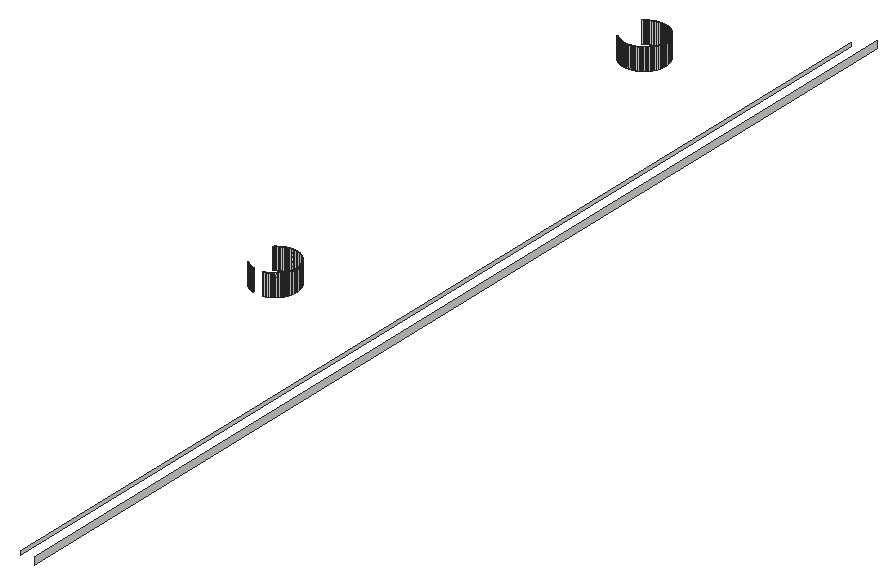
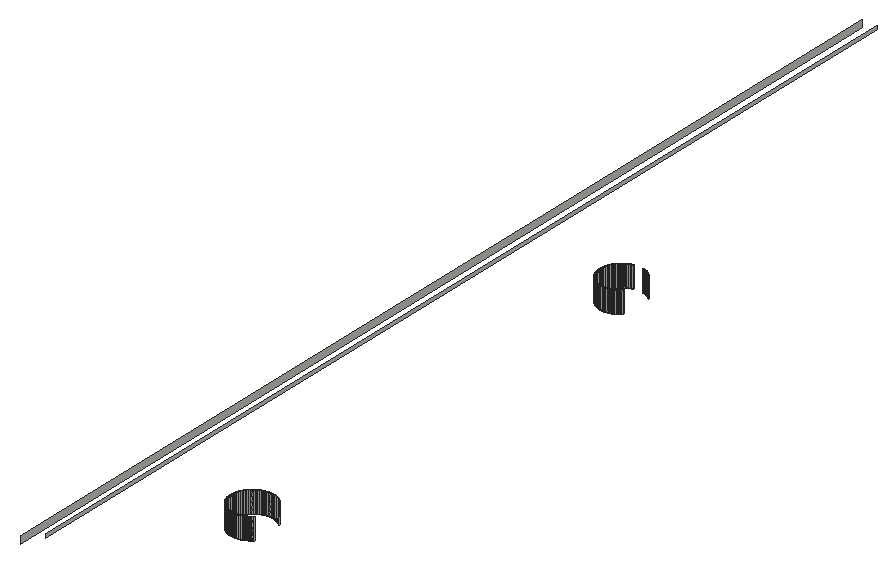
# SketchUp Ruby script. Lengths in inches.
U = 1.inch
M = Sketchup.active_model
def pt(a) = Geom::Point3d.new(a.map { |v| v * U })
def face(e, loops, mat)
  f = e.add_face(loops[0].map { |a| pt(a) })
  loops[1..].each { |l| e.add_face(l.map { |a| pt(a) }).erase! }
  f.material = f.back_material = mat if mat
  f
end
# faces: each face lists its corners as indices into pts; further lists are holes
def faces(e, pts, list, mat = nil) = list.each { |f| face(e, (f[0].is_a?(Array) ? f : [f]).map { |l| l.map { |i| pts[i] } }, mat) }
# xy, xz, yz: faces in a plane at the given z, y or x. An outline is a flat list of corners, or four numbers for a rectangle; further outlines are holes
def ring(l) = l.size == 4 ? [[l[0], l[1]], [l[2], l[1]], [l[2], l[3]], [l[0], l[3]]] : l.each_slice(2).to_a
def flat(e, list, mat, &to3) = list.each { |f| face(e, (f[0].is_a?(Array) ? f : [f]).map { |l| ring(l).map { |u, v| to3.(u, v) } }, mat) }
def xy(e, z, list, mat = nil) = flat(e, list, mat) { |x, y| [x, y, z] }
def xz(e, y, list, mat = nil) = flat(e, list, mat) { |x, z| [x, y, z] }
def yz(e, x, list, mat = nil) = flat(e, list, mat) { |y, z| [x, y, z] }
def lines(e, pts, list) = list.each { |a, b| e.add_line(pt(pts[a]), pt(pts[b])) }
# prism: a flat outline (further loops are holes) pulled along v
def prism(e, loops, v, mat = nil)
  f = face(e, loops, mat); d = Geom::Vector3d.new(v.map { |x| x * U })
  f.pushpull(f.normal.samedirection?(d) ? d.length : -d.length)
end
def box(e, o, s, mat = nil) = prism(e, [[o, [o[0] + s[0], o[1], o[2]], [o[0] + s[0], o[1] + s[1], o[2]], [o[0], o[1] + s[1], o[2]]]], [0, 0, s[2]], mat)
def at(x, y, z, deg = 0) = Geom::Transformation.translation(pt([x, y, z])) * Geom::Transformation.rotation(ORIGIN, Z_AXIS, deg.degrees)
def axes(o, x, y, z) = Geom::Transformation.new([*x, 0, *y, 0, *z, 0, *pt(o).to_a, 1])
def part(name) = M.definitions.add(name)
# library, detail: a bought-in or finely detailed component or shape, given as its bounding box
def library(name, o, s) = part(name).tap { |d| box(d.entities, o, s) }
def detail(e, o, s) = box(e.add_group.entities, o, s)
def put(e, d, t, mat = nil) = e.add_instance(d, t).tap { |i| i.material = mat if mat }
def group(e, t, mat = nil) = e.add_group.tap { |g| g.transformation = t; g.material = mat if mat }.entities
root = M.entities
xz(root,255.5,[[328.84,108,328.92,111],[328.92,108,329,111],[329,108,329.08,111],[329.08,108,329.16,111]])
xz(root,314,[[328.84,108,328.92,111],[328.92,108,329,111],[329,108,329.08,111],[329.08,108,329.16,111]])
xz(root,320,[[328.84,108,328.92,111],[328.92,108,329,111],[329,108,329.08,111],[329.08,108,329.16,111]])
yz(root,332,[[252.34,108,252.42,111],[252.42,108,252.5,111],[252.5,108,252.58,111],[252.58,108,252.66,111],[316.84,108,316.92,111],
  [316.92,108,317,111],[317,108,317.08,111],[317.08,108,317.16,111]])
yz(root,345,[[187.96,108,333,108.5]])
yz(root,347,[[187.97,107.5,335,108.5]])
p = [[328.07,249.65,108],[328,249.67,108],[328,249.67,111],[328.07,249.65,111],[328.15,249.625,108],[328.15,249.625,111],
  [328.22,249.6,108],[328.22,249.6,111],[328.3,249.58,108],[328.3,249.58,111],[328.375,249.57,108],[328.375,249.57,111],
  [329.625,249.57,108],[329.55,249.55,108],[329.55,249.55,111],[329.625,249.57,111],[329.7,249.58,108],[329.7,249.58,111],
  [329.78,249.6,108],[329.78,249.6,111],[329.85,249.625,108],[329.85,249.625,111],[329.93,249.65,108],[329.93,249.65,111],
  [330,249.67,108],[330,249.67,111],[327.85,249.73,108],[327.78,249.76,108],[327.78,249.76,111],[327.85,249.73,111],
  [327.92,249.7,108],[327.92,249.7,111],[330.08,249.7,108],[330.08,249.7,111],[330.15,249.73,108],[330.15,249.73,111],
  [330.22,249.76,108],[330.22,249.76,111],[327.64,249.83,108],[327.57,249.86,108],[327.57,249.86,111],[327.64,249.83,111],
  [327.71,249.79,108],[327.71,249.79,111],[330.29,249.79,108],[330.29,249.79,111],[330.36,249.83,108],[330.36,249.83,111],
  [330.43,249.86,108],[330.43,249.86,111],[327.43,249.94,108],[327.37,249.98,108],[327.37,249.98,111],[327.43,249.94,111],
  [327.5,249.9,108],[327.5,249.9,111],[330.5,249.9,108],[330.5,249.9,111],[330.57,249.94,108],[330.57,249.94,111],
  [330.63,249.98,108],[330.63,249.98,111],[327.3,250.03,108],[327.24,250.07,108],[327.24,250.07,111],[327.3,250.03,111],
  [330.7,250.03,108],[330.7,250.03,111],[330.76,250.07,108],[330.76,250.07,111],[327.17,250.12,108],[327.11,250.17,108],
  [327.11,250.17,111],[327.17,250.12,111],[330.83,250.12,108],[330.83,250.12,111],[330.89,250.17,108],[330.89,250.17,111],
  [327.05,250.22,108],[326.99,250.27,108],[326.99,250.27,111],[327.05,250.22,111],[330.95,250.22,108],[330.95,250.22,111],
  [331.01,250.27,108],[331.01,250.27,111],[326.93,250.32,108],[326.93,250.32,111],[331.07,250.32,108],[331.07,250.32,111],
  [331.12,250.38,108],[331.12,250.38,111],[331.18,250.43,108],[331.18,250.43,111],[331.23,250.49,108],[331.23,250.49,111],
  [331.28,250.55,108],[331.28,250.55,111],[331.33,250.61,108],[331.33,250.61,111],[331.38,250.67,108],[331.38,250.67,111],
  [331.43,250.74,108],[331.43,250.74,111],[331.47,250.8,108],[331.47,250.8,111],[331.52,250.87,108],[331.52,250.87,111],
  [331.56,250.93,108],[331.56,250.93,111],[331.6,251,108],[331.6,251,111],[331.64,251.07,108],[331.64,251.07,111],
  [331.67,251.14,108],[331.67,251.14,111],[331.71,251.21,108],[331.71,251.21,111],[331.74,251.28,108],[331.74,251.28,111],
  [331.77,251.35,108],[331.77,251.35,111],[331.8,251.42,108],[331.8,251.42,111],[331.83,251.5,108],[331.83,251.5,111],
  [331.85,251.57,108],[331.85,251.57,111],[331.875,251.65,108],[331.875,251.65,111],[331.9,251.72,108],[331.9,251.72,111],
  [331.92,251.8,108],[331.92,251.8,111],[331.93,251.875,108],[331.93,251.875,111],[331.95,251.95,108],[331.95,251.95,111],
  [331.96,252.03,108],[331.96,252.03,111],[331.97,252.11,108],[331.97,252.11,111],[331.98,252.1875,108],[331.98,252.1875,111],
  [331.99,252.26,108],[331.99,252.26,111],[332,252.34,108],[332,252.34,111],[331.98,252.8125,108],[331.99,252.74,108],
  [331.99,252.74,111],[331.98,252.8125,111],[332,252.66,108],[332,252.66,111],[331.97,252.89,108],[331.97,252.89,111],
  [331.96,252.97,108],[331.96,252.97,111],[331.93,253.125,108],[331.95,253.05,108],[331.95,253.05,111],[331.93,253.125,111],
  [331.92,253.2,108],[331.92,253.2,111],[331.9,253.28,108],[331.9,253.28,111],[331.875,253.35,108],[331.875,253.35,111],
  [331.83,253.5,108],[331.85,253.43,108],[331.85,253.43,111],[331.83,253.5,111],[331.8,253.58,108],[331.8,253.58,111],
  [331.74,253.72,108],[331.77,253.65,108],[331.77,253.65,111],[331.74,253.72,111],[331.71,253.79,108],[331.71,253.79,111],
  [331.67,253.86,108],[331.67,253.86,111],[331.6,254,108],[331.64,253.93,108],[331.64,253.93,111],[331.6,254,111],
  [331.56,254.07,108],[331.56,254.07,111],[331.47,254.2,108],[331.52,254.13,108],[331.52,254.13,111],[331.47,254.2,111],
  [331.43,254.26,108],[331.43,254.26,111],[331.33,254.39,108],[331.38,254.33,108],[331.38,254.33,111],[331.33,254.39,111],
  [331.23,254.51,108],[331.28,254.45,108],[331.28,254.45,111],[331.23,254.51,111],[331.18,254.57,108],[331.18,254.57,111],
  [331.07,254.68,108],[331.12,254.62,108],[331.12,254.62,111],[331.07,254.68,111],[326.93,254.68,108],[326.99,254.73,108],
  [326.99,254.73,111],[326.93,254.68,111],[327.05,254.78,108],[327.05,254.78,111],[330.95,254.78,108],[331.01,254.73,108],
  [331.01,254.73,111],[330.95,254.78,111],[327.11,254.83,108],[327.11,254.83,111],[327.17,254.88,108],[327.17,254.88,111],
  [330.83,254.88,108],[330.89,254.83,108],[330.89,254.83,111],[330.83,254.88,111],[327.24,254.93,108],[327.24,254.93,111],
  [327.3,254.97,108],[327.3,254.97,111],[330.7,254.97,108],[330.76,254.93,108],[330.76,254.93,111],[330.7,254.97,111],
  [327.37,255.02,108],[327.37,255.02,111],[327.43,255.06,108],[327.43,255.06,111],[330.57,255.06,108],[330.63,255.02,108],
  [330.63,255.02,111],[330.57,255.06,111],[327.5,255.1,108],[327.5,255.1,111],[327.57,255.14,108],[327.57,255.14,111],
  [327.64,255.17,108],[327.64,255.17,111],[330.36,255.17,108],[330.43,255.14,108],[330.43,255.14,111],[330.36,255.17,111],
  [330.5,255.1,108],[330.5,255.1,111],[327.71,255.21,108],[327.71,255.21,111],[327.78,255.24,108],[327.78,255.24,111],
  [327.85,255.27,108],[327.85,255.27,111],[330.15,255.27,108],[330.22,255.24,108],[330.22,255.24,111],[330.15,255.27,111],
  [330.29,255.21,108],[330.29,255.21,111],[327.92,255.3,108],[327.92,255.3,111],[328,255.33,108],[328,255.33,111],
  [328.07,255.35,108],[328.07,255.35,111],[329.93,255.35,108],[330,255.33,108],[330,255.33,111],[329.93,255.35,111],
  [330.08,255.3,108],[330.08,255.3,111],[328.15,255.375,108],[328.15,255.375,111],[328.22,255.4,108],[328.22,255.4,111],
  [328.3,255.42,108],[328.3,255.42,111],[328.375,255.43,108],[328.375,255.43,111],[328.45,255.45,108],[328.45,255.45,111],
  [328.53,255.46,108],[328.53,255.46,111],[329.47,255.46,108],[329.55,255.45,108],[329.55,255.45,111],[329.47,255.46,111],
  [329.625,255.43,108],[329.625,255.43,111],[329.7,255.42,108],[329.7,255.42,111],[329.78,255.4,108],[329.78,255.4,111],
  [329.85,255.375,108],[329.85,255.375,111],[328.61,255.47,108],[328.61,255.47,111],[328.6875,255.48,108],[328.6875,255.48,111],
  [328.76,255.49,108],[328.76,255.49,111],[328.84,255.5,108],[328.84,255.5,111],[329.16,255.5,108],[329.24,255.49,108],
  [329.24,255.49,111],[329.16,255.5,111],[329.3125,255.48,108],[329.3125,255.48,111],[329.39,255.47,108],[329.39,255.47,111],
  [328.53,314.04,108],[328.45,314.05,108],[328.45,314.05,111],[328.53,314.04,111],[328.61,314.03,108],[328.61,314.03,111],
  [328.6875,314.02,108],[328.6875,314.02,111],[328.76,314.01,108],[328.76,314.01,111],[328.84,314,108],[328.84,314,111],
  [329.24,314.01,108],[329.16,314,108],[329.16,314,111],[329.24,314.01,111],[329.3125,314.02,108],[329.3125,314.02,111],
  [329.39,314.03,108],[329.39,314.03,111],[329.47,314.04,108],[329.47,314.04,111],[329.55,314.05,108],[329.55,314.05,111],
  [328.07,314.15,108],[328,314.17,108],[328,314.17,111],[328.07,314.15,111],[328.15,314.125,108],[328.15,314.125,111],
  [328.22,314.1,108],[328.22,314.1,111],[328.3,314.08,108],[328.3,314.08,111],[328.375,314.07,108],[328.375,314.07,111],
  [329.625,314.07,108],[329.625,314.07,111],[329.7,314.08,108],[329.7,314.08,111],[329.78,314.1,108],[329.78,314.1,111],
  [329.85,314.125,108],[329.85,314.125,111],[329.93,314.15,108],[329.93,314.15,111],[330,314.17,108],[330,314.17,111],
  [327.85,314.23,108],[327.78,314.26,108],[327.78,314.26,111],[327.85,314.23,111],[327.92,314.2,108],[327.92,314.2,111],
  [330.08,314.2,108],[330.08,314.2,111],[330.15,314.23,108],[330.15,314.23,111],[330.22,314.26,108],[330.22,314.26,111],
  [327.64,314.33,108],[327.57,314.36,108],[327.57,314.36,111],[327.64,314.33,111],[327.71,314.29,108],[327.71,314.29,111],
  [330.29,314.29,108],[330.29,314.29,111],[330.36,314.33,108],[330.36,314.33,111],[330.43,314.36,108],[330.43,314.36,111],
  [327.43,314.44,108],[327.37,314.48,108],[327.37,314.48,111],[327.43,314.44,111],[327.5,314.4,108],[327.5,314.4,111],
  [330.5,314.4,108],[330.5,314.4,111],[330.57,314.44,108],[330.57,314.44,111],[330.63,314.48,108],[330.63,314.48,111],
  [327.3,314.53,108],[327.24,314.57,108],[327.24,314.57,111],[327.3,314.53,111],[330.7,314.53,108],[330.7,314.53,111],
  [330.76,314.57,108],[330.76,314.57,111],[327.17,314.62,108],[327.11,314.67,108],[327.11,314.67,111],[327.17,314.62,111],
  [330.83,314.62,108],[330.83,314.62,111],[330.89,314.67,108],[330.89,314.67,111],[327.05,314.72,108],[326.99,314.77,108],
  [326.99,314.77,111],[327.05,314.72,111],[330.95,314.72,108],[330.95,314.72,111],[331.01,314.77,108],[331.01,314.77,111],
  [326.93,314.82,108],[326.93,314.82,111],[331.07,314.82,108],[331.07,314.82,111],[331.12,314.88,108],[331.12,314.88,111],
  [331.18,314.93,108],[331.18,314.93,111],[331.23,314.99,108],[331.23,314.99,111],[331.28,315.05,108],[331.28,315.05,111],
  [331.33,315.11,108],[331.33,315.11,111],[331.38,315.17,108],[331.38,315.17,111],[331.43,315.24,108],[331.43,315.24,111],
  [331.47,315.3,108],[331.47,315.3,111],[331.52,315.37,108],[331.52,315.37,111],[331.56,315.43,108],[331.56,315.43,111],
  [331.6,315.5,108],[331.6,315.5,111],[331.64,315.57,108],[331.64,315.57,111],[331.67,315.64,108],[331.67,315.64,111],
  [331.71,315.71,108],[331.71,315.71,111],[331.74,315.78,108],[331.74,315.78,111],[331.77,315.85,108],[331.77,315.85,111],
  [331.8,315.92,108],[331.8,315.92,111],[331.83,316,108],[331.83,316,111],[331.85,316.07,108],[331.85,316.07,111],
  [331.875,316.15,108],[331.875,316.15,111],[331.9,316.22,108],[331.9,316.22,111],[331.92,316.3,108],[331.92,316.3,111],
  [331.93,316.375,108],[331.93,316.375,111],[331.95,316.45,108],[331.95,316.45,111],[331.96,316.53,108],[331.96,316.53,111],
  [331.97,316.61,108],[331.97,316.61,111],[331.98,316.6875,108],[331.98,316.6875,111],[331.99,316.76,108],[331.99,316.76,111],
  [332,316.84,108],[332,316.84,111],[331.98,317.3125,108],[331.99,317.24,108],[331.99,317.24,111],[331.98,317.3125,111],
  [332,317.16,108],[332,317.16,111],[331.97,317.39,108],[331.97,317.39,111],[331.96,317.47,108],[331.96,317.47,111],
  [331.93,317.625,108],[331.95,317.55,108],[331.95,317.55,111],[331.93,317.625,111],[331.92,317.7,108],[331.92,317.7,111],
  [331.9,317.78,108],[331.9,317.78,111],[331.875,317.85,108],[331.875,317.85,111],[331.83,318,108],[331.85,317.93,108],
  [331.85,317.93,111],[331.83,318,111],[331.8,318.08,108],[331.8,318.08,111],[331.74,318.22,108],[331.77,318.15,108],
  [331.77,318.15,111],[331.74,318.22,111],[331.71,318.29,108],[331.71,318.29,111],[331.67,318.36,108],[331.67,318.36,111],
  [331.6,318.5,108],[331.64,318.43,108],[331.64,318.43,111],[331.6,318.5,111],[331.56,318.57,108],[331.56,318.57,111],
  [331.47,318.7,108],[331.52,318.63,108],[331.52,318.63,111],[331.47,318.7,111],[331.43,318.76,108],[331.43,318.76,111],
  [331.33,318.89,108],[331.38,318.83,108],[331.38,318.83,111],[331.33,318.89,111],[331.23,319.01,108],[331.28,318.95,108],
  [331.28,318.95,111],[331.23,319.01,111],[331.18,319.07,108],[331.18,319.07,111],[331.07,319.18,108],[331.12,319.12,108],
  [331.12,319.12,111],[331.07,319.18,111],[326.93,319.18,108],[326.99,319.23,108],[326.99,319.23,111],[326.93,319.18,111],
  [327.05,319.28,108],[327.05,319.28,111],[330.95,319.28,108],[331.01,319.23,108],[331.01,319.23,111],[330.95,319.28,111],
  [327.11,319.33,108],[327.11,319.33,111],[327.17,319.38,108],[327.17,319.38,111],[330.83,319.38,108],[330.89,319.33,108],
  [330.89,319.33,111],[330.83,319.38,111],[327.24,319.43,108],[327.24,319.43,111],[327.3,319.47,108],[327.3,319.47,111],
  [330.7,319.47,108],[330.76,319.43,108],[330.76,319.43,111],[330.7,319.47,111],[327.37,319.52,108],[327.37,319.52,111],
  [327.43,319.56,108],[327.43,319.56,111],[330.57,319.56,108],[330.63,319.52,108],[330.63,319.52,111],[330.57,319.56,111],
  [327.5,319.6,108],[327.5,319.6,111],[327.57,319.64,108],[327.57,319.64,111],[327.64,319.67,108],[327.64,319.67,111],
  [330.36,319.67,108],[330.43,319.64,108],[330.43,319.64,111],[330.36,319.67,111],[330.5,319.6,108],[330.5,319.6,111],
  [327.71,319.71,108],[327.71,319.71,111],[327.78,319.74,108],[327.78,319.74,111],[327.85,319.77,108],[327.85,319.77,111],
  [330.15,319.77,108],[330.22,319.74,108],[330.22,319.74,111],[330.15,319.77,111],[330.29,319.71,108],[330.29,319.71,111],
  [327.92,319.8,108],[327.92,319.8,111],[328,319.83,108],[328,319.83,111],[328.07,319.85,108],[328.07,319.85,111],
  [329.93,319.85,108],[330,319.83,108],[330,319.83,111],[329.93,319.85,111],[330.08,319.8,108],[330.08,319.8,111],
  [328.15,319.875,108],[328.15,319.875,111],[328.22,319.9,108],[328.22,319.9,111],[328.3,319.92,108],[328.3,319.92,111],
  [328.375,319.93,108],[328.375,319.93,111],[328.45,319.95,108],[328.45,319.95,111],[328.53,319.96,108],[328.53,319.96,111],
  [329.47,319.96,108],[329.55,319.95,108],[329.55,319.95,111],[329.47,319.96,111],[329.625,319.93,108],[329.625,319.93,111],
  [329.7,319.92,108],[329.7,319.92,111],[329.78,319.9,108],[329.78,319.9,111],[329.85,319.875,108],[329.85,319.875,111],
  [328.61,319.97,108],[328.61,319.97,111],[328.6875,319.98,108],[328.6875,319.98,111],[328.76,319.99,108],[328.76,319.99,111],
  [328.84,320,108],[328.84,320,111],[329.16,320,108],[329.24,319.99,108],[329.24,319.99,111],[329.16,320,111],
  [329.3125,319.98,108],[329.3125,319.98,111],[329.39,319.97,108],[329.39,319.97,111]]
faces(root,p,[[0,1,2,3],[4,0,3,5],[6,4,5,7],[8,6,7,9],[10,8,9,11],[12,13,14,15],[16,12,15,17],[18,16,17,19],
  [20,18,19,21],[22,20,21,23],[24,22,23,25],[26,27,28,29],[30,26,29,31],[1,30,31,2],[32,24,25,33],[34,32,33,35],
  [36,34,35,37],[38,39,40,41],[42,38,41,43],[27,42,43,28],[44,36,37,45],[46,44,45,47],[48,46,47,49],[50,51,52,53],
  [54,50,53,55],[39,54,55,40],[56,48,49,57],[58,56,57,59],[60,58,59,61],[62,63,64,65],[51,62,65,52],[66,60,61,67],
  [68,66,67,69],[70,71,72,73],[63,70,73,64],[74,68,69,75],[76,74,75,77],[78,79,80,81],[71,78,81,72],[82,76,77,83],
  [84,82,83,85],[79,86,87,80],[88,84,85,89],[90,88,89,91],[92,90,91,93],[94,92,93,95],[96,94,95,97],[98,96,97,99],
  [100,98,99,101],[102,100,101,103],[104,102,103,105],[106,104,105,107],[108,106,107,109],[110,108,109,111],[112,110,111,113],[114,112,113,115],
  [116,114,115,117],[118,116,117,119],[120,118,119,121],[122,120,121,123],[124,122,123,125],[126,124,125,127],[128,126,127,129],[130,128,129,131],
  [132,130,131,133],[134,132,133,135],[136,134,135,137],[138,136,137,139],[140,138,139,141],[142,140,141,143],[144,142,143,145],[146,144,145,147],
  [148,149,150,151],[149,152,153,150],[154,148,151,155],[156,154,155,157],[158,159,160,161],[159,156,157,160],[162,158,161,163],[164,162,163,165],
  [166,164,165,167],[168,169,170,171],[169,166,167,170],[172,168,171,173],[174,175,176,177],[175,172,173,176],[178,174,177,179],[180,178,179,181],
  [182,183,184,185],[183,180,181,184],[186,182,185,187],[188,189,190,191],[189,186,187,190],[192,188,191,193],[194,195,196,197],[195,192,193,196],
  [198,199,200,201],[199,194,197,200],[202,198,201,203],[204,205,206,207],[205,202,203,206],[208,209,210,211],[209,212,213,210],[214,215,216,217],
  [215,204,207,216],[212,218,219,213],[218,220,221,219],[222,223,224,225],[223,214,217,224],[220,226,227,221],[226,228,229,227],[230,231,232,233],
  [231,222,225,232],[228,234,235,229],[234,236,237,235],[238,239,240,241],[239,230,233,240],[236,242,243,237],[242,244,245,243],[244,246,247,245],
  [248,249,250,251],[249,252,253,250],[252,238,241,253],[246,254,255,247],[254,256,257,255],[256,258,259,257],[260,261,262,263],[261,264,265,262],
  [264,248,251,265],[258,266,267,259],[266,268,269,267],[268,270,271,269],[272,273,274,275],[273,276,277,274],[276,260,263,277],[270,278,279,271],
  [278,280,281,279],[280,282,283,281],[282,284,285,283],[284,286,287,285],[286,288,289,287],[290,291,292,293],[291,294,295,292],[294,296,297,295],
  [296,298,299,297],[298,300,301,299],[300,272,275,301],[288,302,303,289],[302,304,305,303],[304,306,307,305],[306,308,309,307],[310,311,312,313],
  [311,314,315,312],[314,316,317,315],[316,290,293,317],[318,319,320,321],[322,318,321,323],[324,322,323,325],[326,324,325,327],[328,326,327,329],
  [330,331,332,333],[334,330,333,335],[336,334,335,337],[338,336,337,339],[340,338,339,341],[342,343,344,345],[346,342,345,347],[348,346,347,349],
  [350,348,349,351],[352,350,351,353],[319,352,353,320],[354,340,341,355],[356,354,355,357],[358,356,357,359],[360,358,359,361],[362,360,361,363],
  [364,362,363,365],[366,367,368,369],[370,366,369,371],[343,370,371,344],[372,364,365,373],[374,372,373,375],[376,374,375,377],[378,379,380,381],
  [382,378,381,383],[367,382,383,368],[384,376,377,385],[386,384,385,387],[388,386,387,389],[390,391,392,393],[394,390,393,395],[379,394,395,380],
  [396,388,389,397],[398,396,397,399],[400,398,399,401],[402,403,404,405],[391,402,405,392],[406,400,401,407],[408,406,407,409],[410,411,412,413],
  [403,410,413,404],[414,408,409,415],[416,414,415,417],[418,419,420,421],[411,418,421,412],[422,416,417,423],[424,422,423,425],[419,426,427,420],
  [428,424,425,429],[430,428,429,431],[432,430,431,433],[434,432,433,435],[436,434,435,437],[438,436,437,439],[440,438,439,441],[442,440,441,443],
  [444,442,443,445],[446,444,445,447],[448,446,447,449],[450,448,449,451],[452,450,451,453],[454,452,453,455],[456,454,455,457],[458,456,457,459],
  [460,458,459,461],[462,460,461,463],[464,462,463,465],[466,464,465,467],[468,466,467,469],[470,468,469,471],[472,470,471,473],[474,472,473,475],
  [476,474,475,477],[478,476,477,479],[480,478,479,481],[482,480,481,483],[484,482,483,485],[486,484,485,487],[488,489,490,491],[489,492,493,490],
  [494,488,491,495],[496,494,495,497],[498,499,500,501],[499,496,497,500],[502,498,501,503],[504,502,503,505],[506,504,505,507],[508,509,510,511],
  [509,506,507,510],[512,508,511,513],[514,515,516,517],[515,512,513,516],[518,514,517,519],[520,518,519,521],[522,523,524,525],[523,520,521,524],
  [526,522,525,527],[528,529,530,531],[529,526,527,530],[532,528,531,533],[534,535,536,537],[535,532,533,536],[538,539,540,541],[539,534,537,540],
  [542,538,541,543],[544,545,546,547],[545,542,543,546],[548,549,550,551],[549,552,553,550],[554,555,556,557],[555,544,547,556],[552,558,559,553],
  [558,560,561,559],[562,563,564,565],[563,554,557,564],[560,566,567,561],[566,568,569,567],[570,571,572,573],[571,562,565,572],[568,574,575,569],
  [574,576,577,575],[578,579,580,581],[579,570,573,580],[576,582,583,577],[582,584,585,583],[584,586,587,585],[588,589,590,591],[589,592,593,590],
  [592,578,581,593],[586,594,595,587],[594,596,597,595],[596,598,599,597],[600,601,602,603],[601,604,605,602],[604,588,591,605],[598,606,607,599],
  [606,608,609,607],[608,610,611,609],[612,613,614,615],[613,616,617,614],[616,600,603,617],[610,618,619,611],[618,620,621,619],[620,622,623,621],
  [622,624,625,623],[624,626,627,625],[626,628,629,627],[630,631,632,633],[631,634,635,632],[634,636,637,635],[636,638,639,637],[638,640,641,639],
  [640,612,615,641],[628,642,643,629],[642,644,645,643],[644,646,647,645],[646,648,649,647],[650,651,652,653],[651,654,655,652],[654,656,657,655],
  [656,630,633,657]])
